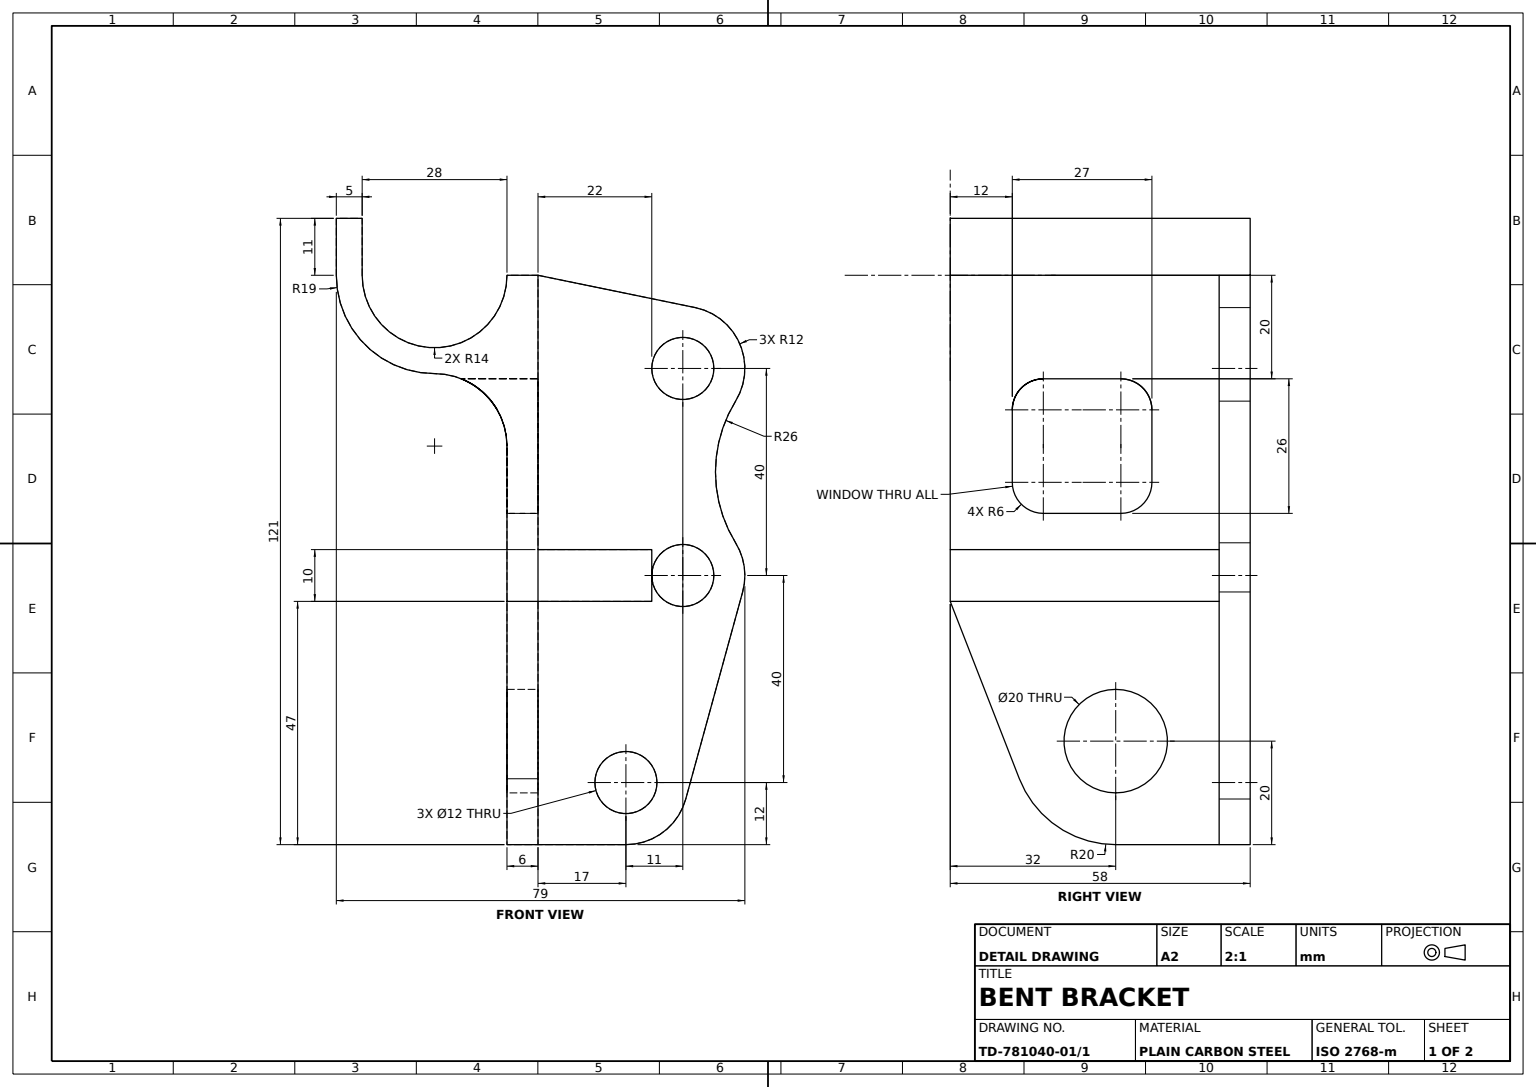
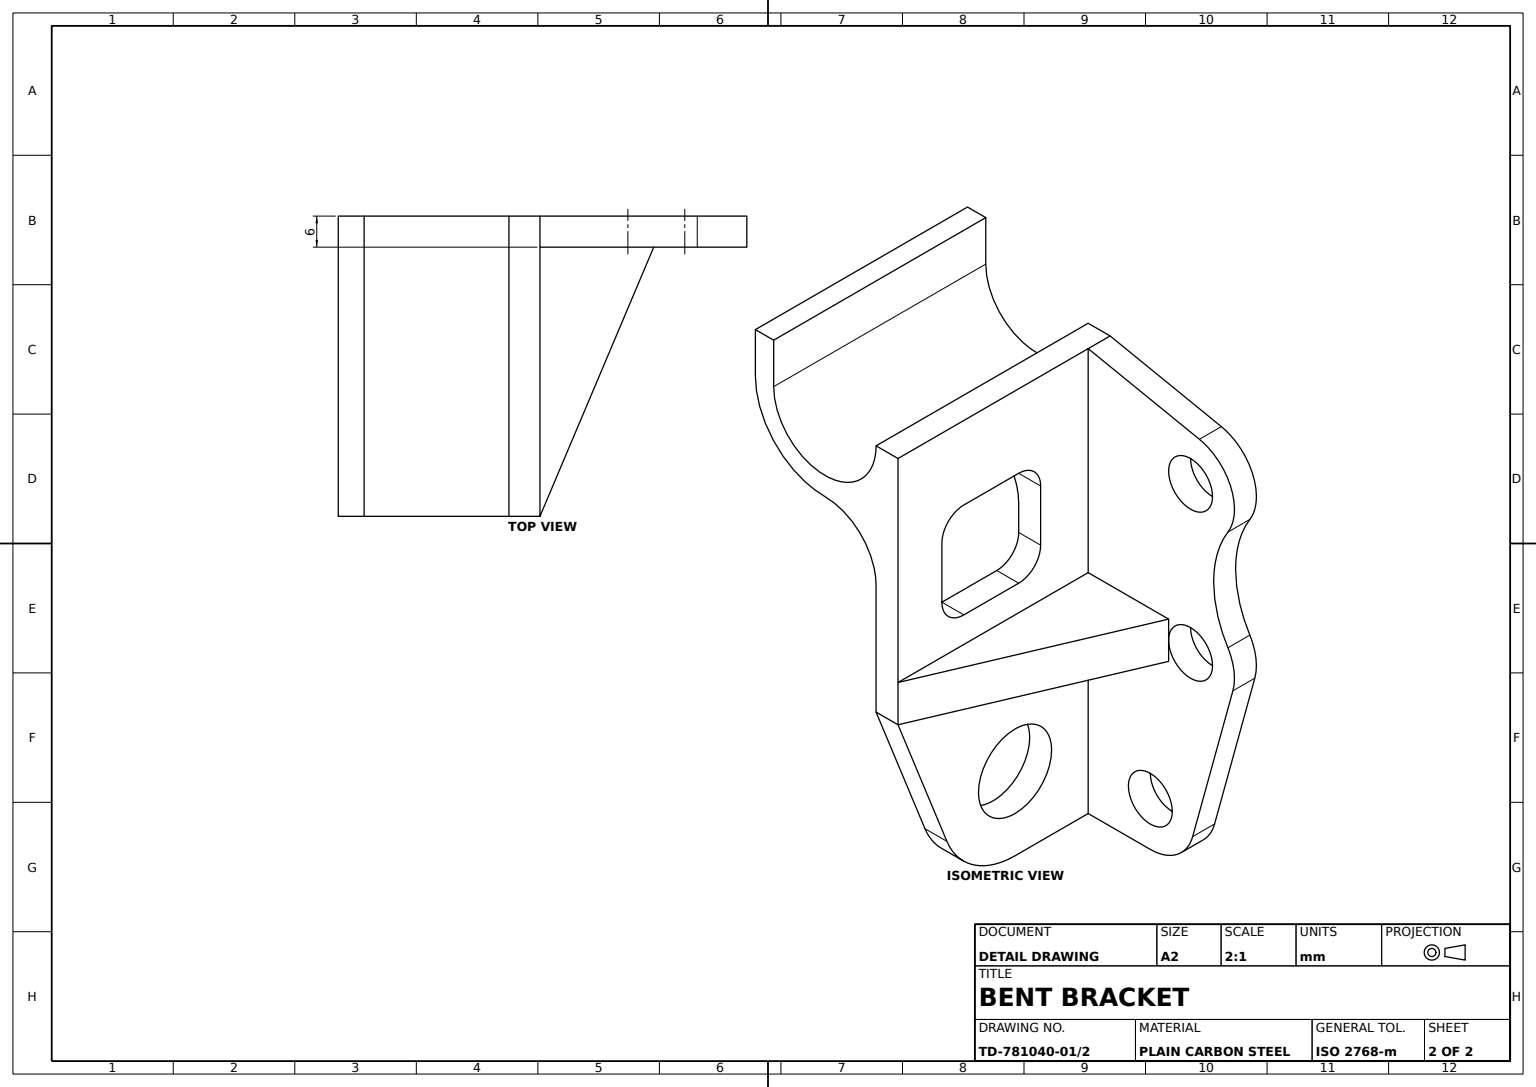
ISO-10303-21;
HEADER;
FILE_DESCRIPTION((''),'2;1');
FILE_NAME('','',(''),(''),'','','');
FILE_SCHEMA(('AUTOMOTIVE_DESIGN'));
ENDSEC;
DATA;
#1=APPLICATION_CONTEXT('');
#2=PRODUCT_CONTEXT('',#1,'mechanical');
#3=PRODUCT('','','',(#2));
#4=PRODUCT_DEFINITION_FORMATION('','',#3);
#5=PRODUCT_DEFINITION_CONTEXT('',#1,'design');
#6=PRODUCT_DEFINITION('','',#4,#5);
#7=PRODUCT_DEFINITION_SHAPE('','',#6);
#8=(LENGTH_UNIT()NAMED_UNIT(*)SI_UNIT(.MILLI.,.METRE.));
#9=(NAMED_UNIT(*)PLANE_ANGLE_UNIT()SI_UNIT($,.RADIAN.));
#10=(NAMED_UNIT(*)SI_UNIT($,.STERADIAN.)SOLID_ANGLE_UNIT());
#11=UNCERTAINTY_MEASURE_WITH_UNIT(LENGTH_MEASURE(1.E-05),#8,'distance_accuracy_value','');
#12=(GEOMETRIC_REPRESENTATION_CONTEXT(3)GLOBAL_UNCERTAINTY_ASSIGNED_CONTEXT((#11))GLOBAL_UNIT_ASSIGNED_CONTEXT((#8,#9,#10))REPRESENTATION_CONTEXT('',''));
#13=CARTESIAN_POINT('',(-39.,69.,-29.));
#14=VERTEX_POINT('',#13);
#15=CARTESIAN_POINT('',(-39.,58.,-29.));
#16=VERTEX_POINT('',#15);
#17=CARTESIAN_POINT('',(-39.,0.,-29.));
#18=DIRECTION('',(0.,-1.,0.));
#19=VECTOR('',#18,1000.);
#20=LINE('',#17,#19);
#21=EDGE_CURVE('',#14,#16,#20,.T.);
#22=ORIENTED_EDGE('',*,*,#21,.T.);
#23=CARTESIAN_POINT('',(-39.,58.,29.));
#24=VERTEX_POINT('',#23);
#25=DIRECTION('',(0.,0.,-1.));
#26=VECTOR('',#25,1000.);
#27=LINE('',#23,#26);
#28=EDGE_CURVE('',#24,#16,#27,.T.);
#29=ORIENTED_EDGE('',*,*,#28,.F.);
#30=CARTESIAN_POINT('',(-39.,69.,29.));
#31=VERTEX_POINT('',#30);
#32=CARTESIAN_POINT('',(-39.,0.,29.));
#33=LINE('',#32,#19);
#34=EDGE_CURVE('',#31,#24,#33,.T.);
#35=ORIENTED_EDGE('',*,*,#34,.F.);
#36=LINE('',#30,#26);
#37=EDGE_CURVE('',#31,#14,#36,.T.);
#38=ORIENTED_EDGE('',*,*,#37,.T.);
#39=EDGE_LOOP('',(#22,#29,#35,#38));
#40=FACE_OUTER_BOUND('',#39,.T.);
#41=DIRECTION('',(1.,0.,0.));
#42=DIRECTION('',(0.,1.,0.));
#43=AXIS2_PLACEMENT_3D('',#32,#41,#42);
#44=PLANE('',#43);
#45=ADVANCED_FACE('',(#40),#44,.F.);
#46=CARTESIAN_POINT('',(0.,-42.,-3.));
#47=VERTEX_POINT('',#46);
#48=CARTESIAN_POINT('',(0.,-22.,-3.));
#49=VERTEX_POINT('',#48);
#50=CARTESIAN_POINT('',(0.,-32.,-3.));
#51=AXIS2_PLACEMENT_3D('',#50,#41,#42);
#52=CIRCLE('',#51,10.);
#53=EDGE_CURVE('',#47,#49,#52,.T.);
#54=ORIENTED_EDGE('',*,*,#53,.F.);
#55=EDGE_CURVE('',#49,#47,#52,.T.);
#56=ORIENTED_EDGE('',*,*,#55,.F.);
#57=EDGE_LOOP('',(#54,#56));
#58=FACE_BOUND('',#57,.T.);
#59=CARTESIAN_POINT('',(0.,-39.268234,15.632573));
#60=VERTEX_POINT('',#59);
#61=CARTESIAN_POINT('',(0.,-52.,-3.));
#62=VERTEX_POINT('',#61);
#63=CIRCLE('',#51,20.);
#64=EDGE_CURVE('',#60,#62,#63,.T.);
#65=ORIENTED_EDGE('',*,*,#64,.T.);
#66=CARTESIAN_POINT('',(0.,-52.,-23.));
#67=VERTEX_POINT('',#66);
#68=CARTESIAN_POINT('',(0.,-52.,29.));
#69=LINE('',#68,#26);
#70=EDGE_CURVE('',#62,#67,#69,.T.);
#71=ORIENTED_EDGE('',*,*,#70,.T.);
#72=CARTESIAN_POINT('',(0.,-5.,-23.));
#73=VERTEX_POINT('',#72);
#74=CARTESIAN_POINT('',(0.,0.,-23.));
#75=LINE('',#74,#19);
#76=EDGE_CURVE('',#73,#67,#75,.T.);
#77=ORIENTED_EDGE('',*,*,#76,.F.);
#78=CARTESIAN_POINT('',(0.,-5.,29.));
#79=VERTEX_POINT('',#78);
#80=CARTESIAN_POINT('',(0.,-5.,0.));
#81=LINE('',#80,#26);
#82=EDGE_CURVE('',#79,#73,#81,.T.);
#83=ORIENTED_EDGE('',*,*,#82,.F.);
#84=CARTESIAN_POINT('',(0.,-10.478719,26.86285));
#85=DIRECTION('',(0.,0.931628639,0.363411721));
#86=VECTOR('',#85,1000.);
#87=LINE('',#84,#86);
#88=EDGE_CURVE('',#60,#79,#87,.T.);
#89=ORIENTED_EDGE('',*,*,#88,.F.);
#90=EDGE_LOOP('',(#65,#71,#77,#83,#89));
#91=FACE_OUTER_BOUND('',#90,.T.);
#92=CARTESIAN_POINT('',(0.,0.,29.));
#93=AXIS2_PLACEMENT_3D('',#92,#41,#42);
#94=PLANE('',#93);
#95=ADVANCED_FACE('',(#58,#91),#94,.T.);
#96=CARTESIAN_POINT('',(22.,0.,-23.));
#97=VERTEX_POINT('',#96);
#98=CARTESIAN_POINT('',(22.,-5.,-23.));
#99=VERTEX_POINT('',#98);
#100=CARTESIAN_POINT('',(22.,5.,-23.));
#101=LINE('',#100,#19);
#102=EDGE_CURVE('',#97,#99,#101,.T.);
#103=ORIENTED_EDGE('',*,*,#102,.F.);
#104=VERTEX_POINT('',#100);
#105=EDGE_CURVE('',#104,#97,#101,.T.);
#106=ORIENTED_EDGE('',*,*,#105,.F.);
#107=CARTESIAN_POINT('',(0.,5.,29.));
#108=VERTEX_POINT('',#107);
#109=CARTESIAN_POINT('',(10.406524,5.,4.40276));
#110=DIRECTION('',(0.389639991,0.,-0.920967251));
#111=VECTOR('',#110,1000.);
#112=LINE('',#109,#111);
#113=EDGE_CURVE('',#108,#104,#112,.T.);
#114=ORIENTED_EDGE('',*,*,#113,.F.);
#115=LINE('',#107,#19);
#116=EDGE_CURVE('',#108,#79,#115,.T.);
#117=ORIENTED_EDGE('',*,*,#116,.T.);
#118=CARTESIAN_POINT('',(10.406524,-5.,4.40276));
#119=LINE('',#118,#111);
#120=EDGE_CURVE('',#79,#99,#119,.T.);
#121=ORIENTED_EDGE('',*,*,#120,.T.);
#122=EDGE_LOOP('',(#103,#106,#114,#117,#121));
#123=FACE_OUTER_BOUND('',#122,.T.);
#124=DIRECTION('',(-0.920967251,0.,-0.389639991));
#125=DIRECTION('',(-0.389639991,0.,0.920967251));
#126=AXIS2_PLACEMENT_3D('',#109,#124,#125);
#127=PLANE('',#126);
#128=ADVANCED_FACE('',(#123),#127,.F.);
#129=ORIENTED_EDGE('',*,*,#64,.F.);
#130=CARTESIAN_POINT('',(-6.,-39.268234,15.632573));
#131=VERTEX_POINT('',#130);
#132=CARTESIAN_POINT('',(-39.001,-39.268234,15.632573));
#133=VECTOR('',#41,1000.);
#134=LINE('',#132,#133);
#135=EDGE_CURVE('',#131,#60,#134,.T.);
#136=ORIENTED_EDGE('',*,*,#135,.F.);
#137=CARTESIAN_POINT('',(-6.,-52.,-3.));
#138=VERTEX_POINT('',#137);
#139=CARTESIAN_POINT('',(-6.,-32.,-3.));
#140=DIRECTION('',(-1.,0.,0.));
#141=AXIS2_PLACEMENT_3D('',#139,#140,#42);
#142=CIRCLE('',#141,20.);
#143=EDGE_CURVE('',#138,#131,#142,.T.);
#144=ORIENTED_EDGE('',*,*,#143,.F.);
#145=CARTESIAN_POINT('',(-39.001,-52.,-3.));
#146=LINE('',#145,#133);
#147=EDGE_CURVE('',#138,#62,#146,.T.);
#148=ORIENTED_EDGE('',*,*,#147,.T.);
#149=EDGE_LOOP('',(#129,#136,#144,#148));
#150=FACE_OUTER_BOUND('',#149,.T.);
#151=CARTESIAN_POINT('',(-39.001,-32.,-3.));
#152=AXIS2_PLACEMENT_3D('',#151,#41,#42);
#153=CYLINDRICAL_SURFACE('',#152,20.);
#154=ADVANCED_FACE('',(#150),#153,.T.);
#155=CARTESIAN_POINT('',(30.413758,51.754734,-23.));
#156=VERTEX_POINT('',#155);
#157=CARTESIAN_POINT('',(30.413758,51.754734,-29.));
#158=VERTEX_POINT('',#157);
#159=LINE('',#155,#26);
#160=EDGE_CURVE('',#156,#158,#159,.T.);
#161=ORIENTED_EDGE('',*,*,#160,.F.);
#162=CARTESIAN_POINT('',(38.20347,33.684211,-23.));
#163=VERTEX_POINT('',#162);
#164=CARTESIAN_POINT('',(28.,40.,-23.));
#165=DIRECTION('',(0.,0.,1.));
#166=AXIS2_PLACEMENT_3D('',#164,#165,#41);
#167=CIRCLE('',#166,12.);
#168=EDGE_CURVE('',#163,#156,#167,.T.);
#169=ORIENTED_EDGE('',*,*,#168,.F.);
#170=CARTESIAN_POINT('',(38.20347,33.684211,-29.));
#171=VERTEX_POINT('',#170);
#172=LINE('',#162,#26);
#173=EDGE_CURVE('',#163,#171,#172,.T.);
#174=ORIENTED_EDGE('',*,*,#173,.T.);
#175=CARTESIAN_POINT('',(28.,40.,-29.));
#176=AXIS2_PLACEMENT_3D('',#175,#165,#41);
#177=CIRCLE('',#176,12.);
#178=EDGE_CURVE('',#171,#158,#177,.T.);
#179=ORIENTED_EDGE('',*,*,#178,.T.);
#180=EDGE_LOOP('',(#161,#169,#174,#179));
#181=FACE_OUTER_BOUND('',#180,.T.);
#182=AXIS2_PLACEMENT_3D('',#164,#25,#140);
#183=CYLINDRICAL_SURFACE('',#182,12.);
#184=ADVANCED_FACE('',(#181),#183,.T.);
#185=CARTESIAN_POINT('',(0.,58.,29.));
#186=VERTEX_POINT('',#185);
#187=CARTESIAN_POINT('',(-6.,58.,29.));
#188=VERTEX_POINT('',#187);
#189=VECTOR('',#140,1000.);
#190=LINE('',#185,#189);
#191=EDGE_CURVE('',#186,#188,#190,.T.);
#192=ORIENTED_EDGE('',*,*,#191,.F.);
#193=CARTESIAN_POINT('',(0.,58.,-23.));
#194=VERTEX_POINT('',#193);
#195=LINE('',#185,#26);
#196=EDGE_CURVE('',#186,#194,#195,.T.);
#197=ORIENTED_EDGE('',*,*,#196,.T.);
#198=CARTESIAN_POINT('',(0.,58.,-29.));
#199=VERTEX_POINT('',#198);
#200=LINE('',#193,#26);
#201=EDGE_CURVE('',#194,#199,#200,.T.);
#202=ORIENTED_EDGE('',*,*,#201,.T.);
#203=CARTESIAN_POINT('',(-6.,58.,-29.));
#204=VERTEX_POINT('',#203);
#205=LINE('',#198,#189);
#206=EDGE_CURVE('',#199,#204,#205,.T.);
#207=ORIENTED_EDGE('',*,*,#206,.T.);
#208=LINE('',#187,#26);
#209=EDGE_CURVE('',#188,#204,#208,.T.);
#210=ORIENTED_EDGE('',*,*,#209,.F.);
#211=EDGE_LOOP('',(#192,#197,#202,#207,#210));
#212=FACE_OUTER_BOUND('',#211,.T.);
#213=AXIS2_PLACEMENT_3D('',#185,#18,#41);
#214=PLANE('',#213);
#215=ADVANCED_FACE('',(#212),#214,.F.);
#216=CARTESIAN_POINT('',(-20.,39.,29.));
#217=VERTEX_POINT('',#216);
#218=CARTESIAN_POINT('',(-20.,58.,29.));
#219=AXIS2_PLACEMENT_3D('',#218,#165,#41);
#220=CIRCLE('',#219,19.);
#221=EDGE_CURVE('',#24,#217,#220,.T.);
#222=ORIENTED_EDGE('',*,*,#221,.F.);
#223=ORIENTED_EDGE('',*,*,#28,.T.);
#224=CARTESIAN_POINT('',(-20.,39.,-29.));
#225=VERTEX_POINT('',#224);
#226=CARTESIAN_POINT('',(-20.,58.,-29.));
#227=AXIS2_PLACEMENT_3D('',#226,#165,#41);
#228=CIRCLE('',#227,19.);
#229=EDGE_CURVE('',#16,#225,#228,.T.);
#230=ORIENTED_EDGE('',*,*,#229,.T.);
#231=VECTOR('',#165,1000.);
#232=LINE('',#216,#231);
#233=EDGE_CURVE('',#225,#217,#232,.T.);
#234=ORIENTED_EDGE('',*,*,#233,.T.);
#235=EDGE_LOOP('',(#222,#223,#230,#234));
#236=FACE_OUTER_BOUND('',#235,.T.);
#237=AXIS2_PLACEMENT_3D('',#218,#25,#140);
#238=CYLINDRICAL_SURFACE('',#237,19.);
#239=ADVANCED_FACE('',(#236),#238,.T.);
#240=ORIENTED_EDGE('',*,*,#173,.F.);
#241=CARTESIAN_POINT('',(34.310989,20.,-23.));
#242=VERTEX_POINT('',#241);
#243=CARTESIAN_POINT('',(60.310989,20.,-23.));
#244=AXIS2_PLACEMENT_3D('',#243,#165,#41);
#245=CIRCLE('',#244,26.);
#246=EDGE_CURVE('',#163,#242,#245,.T.);
#247=ORIENTED_EDGE('',*,*,#246,.T.);
#248=CARTESIAN_POINT('',(34.310989,20.,-29.));
#249=VERTEX_POINT('',#248);
#250=LINE('',#241,#26);
#251=EDGE_CURVE('',#242,#249,#250,.T.);
#252=ORIENTED_EDGE('',*,*,#251,.T.);
#253=CARTESIAN_POINT('',(60.310989,20.,-29.));
#254=AXIS2_PLACEMENT_3D('',#253,#165,#41);
#255=CIRCLE('',#254,26.);
#256=EDGE_CURVE('',#171,#249,#255,.T.);
#257=ORIENTED_EDGE('',*,*,#256,.F.);
#258=EDGE_LOOP('',(#240,#247,#252,#257));
#259=FACE_OUTER_BOUND('',#258,.T.);
#260=AXIS2_PLACEMENT_3D('',#243,#25,#140);
#261=CYLINDRICAL_SURFACE('',#260,26.);
#262=ADVANCED_FACE('',(#259),#261,.F.);
#263=ORIENTED_EDGE('',*,*,#120,.F.);
#264=ORIENTED_EDGE('',*,*,#82,.T.);
#265=LINE('',#72,#133);
#266=EDGE_CURVE('',#73,#99,#265,.T.);
#267=ORIENTED_EDGE('',*,*,#266,.T.);
#268=EDGE_LOOP('',(#263,#264,#267));
#269=FACE_OUTER_BOUND('',#268,.T.);
#270=AXIS2_PLACEMENT_3D('',#80,#42,#165);
#271=PLANE('',#270);
#272=ADVANCED_FACE('',(#269),#271,.F.);
#273=CARTESIAN_POINT('',(-6.,25.,-10.));
#274=VERTEX_POINT('',#273);
#275=CARTESIAN_POINT('',(-6.,25.,-29.));
#276=VERTEX_POINT('',#275);
#277=LINE('',#275,#26);
#278=EDGE_CURVE('',#274,#276,#277,.T.);
#279=ORIENTED_EDGE('',*,*,#278,.F.);
#280=CARTESIAN_POINT('',(-7.875644,32.,-10.));
#281=VERTEX_POINT('',#280);
#282=CARTESIAN_POINT('',(-20.,25.,-10.));
#283=AXIS2_PLACEMENT_3D('',#282,#25,#42);
#284=CIRCLE('',#283,14.);
#285=EDGE_CURVE('',#281,#274,#284,.T.);
#286=ORIENTED_EDGE('',*,*,#285,.F.);
#287=CARTESIAN_POINT('',(-14.803848,38.,-4.));
#288=VERTEX_POINT('',#287);
#289=CARTESIAN_POINT('',(-8.125276,32.432375,-10.));
#290=CARTESIAN_POINT('',(-8.392507,32.842114,-9.95397));
#291=CARTESIAN_POINT('',(-8.959761,33.622399,-9.790228));
#292=CARTESIAN_POINT('',(-9.259803,33.992885,-9.67229));
#293=CARTESIAN_POINT('',(-9.891376,34.697398,-9.373128));
#294=CARTESIAN_POINT('',(-10.216944,35.024563,-9.194584));
#295=CARTESIAN_POINT('',(-10.876753,35.628565,-8.792201));
#296=CARTESIAN_POINT('',(-11.212374,35.906825,-8.567711));
#297=CARTESIAN_POINT('',(-11.891238,36.420559,-8.072582));
#298=CARTESIAN_POINT('',(-12.236165,36.656785,-7.800557));
#299=CARTESIAN_POINT('',(-12.909548,37.078214,-7.215839));
#300=CARTESIAN_POINT('',(-13.240228,37.265008,-6.902669));
#301=CARTESIAN_POINT('',(-13.710866,37.509117,-6.384549));
#302=CARTESIAN_POINT('',(-13.864124,37.584761,-6.202612));
#303=CARTESIAN_POINT('',(-14.151016,37.720636,-5.820819));
#304=CARTESIAN_POINT('',(-14.284805,37.780965,-5.62123));
#305=CARTESIAN_POINT('',(-14.520473,37.883761,-5.195532));
#306=CARTESIAN_POINT('',(-14.621249,37.925746,-4.970388));
#307=CARTESIAN_POINT('',(-14.762952,37.983805,-4.50019));
#308=CARTESIAN_POINT('',(-14.803848,38.,-4.250793));
#309=B_SPLINE_CURVE_WITH_KNOTS('',3,(#280,#289,#290,#291,#292,#293,#294,#295,#296,#297,#298,#299,#300,#301,#302,#303,#304,#305,#306,#307,#308,#287),.UNSPECIFIED.,.F.,.F.,(4,2,2,2,2,2,2,2,2,2,4),(0.,0.001467721,0.002935441,0.004403162,0.005870883,0.007338603,0.008806324,0.009540185,0.010274045,0.011007905,0.011741766),.UNSPECIFIED.);
#310=EDGE_CURVE('',#281,#288,#309,.T.);
#311=ORIENTED_EDGE('',*,*,#310,.T.);
#312=CARTESIAN_POINT('',(-14.803848,38.,11.));
#313=VERTEX_POINT('',#312);
#314=CARTESIAN_POINT('',(-14.803848,38.,29.));
#315=LINE('',#314,#26);
#316=EDGE_CURVE('',#313,#288,#315,.T.);
#317=ORIENTED_EDGE('',*,*,#316,.F.);
#318=CARTESIAN_POINT('',(-7.875644,32.,17.));
#319=VERTEX_POINT('',#318);
#320=CARTESIAN_POINT('',(-14.803848,38.,11.251475));
#321=CARTESIAN_POINT('',(-14.764237,37.984323,11.494618));
#322=CARTESIAN_POINT('',(-14.657915,37.940773,11.849361));
#323=CARTESIAN_POINT('',(-14.614432,37.922788,11.966237));
#324=CARTESIAN_POINT('',(-14.516975,37.88174,12.190868));
#325=CARTESIAN_POINT('',(-14.462779,37.858587,12.299538));
#326=CARTESIAN_POINT('',(-14.287457,37.78214,12.616849));
#327=CARTESIAN_POINT('',(-14.153234,37.721658,12.817654));
#328=CARTESIAN_POINT('',(-13.865997,37.585677,13.200329));
#329=CARTESIAN_POINT('',(-13.714419,37.510893,13.380397));
#330=CARTESIAN_POINT('',(-13.245627,37.26794,13.897196));
#331=CARTESIAN_POINT('',(-12.91481,37.081351,14.211051));
#332=CARTESIAN_POINT('',(-12.238747,36.658555,14.798531));
#333=CARTESIAN_POINT('',(-11.896553,36.424247,15.06842));
#334=CARTESIAN_POINT('',(-11.220981,35.913665,15.561714));
#335=CARTESIAN_POINT('',(-10.886032,35.636525,15.786171));
#336=CARTESIAN_POINT('',(-10.390731,35.183907,16.088779));
#337=CARTESIAN_POINT('',(-10.226798,35.026854,16.183907));
#338=CARTESIAN_POINT('',(-9.901596,34.699253,16.361789));
#339=CARTESIAN_POINT('',(-9.74014,34.528414,16.444573));
#340=CARTESIAN_POINT('',(-9.26836,34.002974,16.668607));
#341=CARTESIAN_POINT('',(-8.967882,33.632936,16.787409));
#342=CARTESIAN_POINT('',(-8.396921,32.848806,16.95316));
#343=CARTESIAN_POINT('',(-8.124796,32.431543,17.));
#344=B_SPLINE_CURVE_WITH_KNOTS('',3,(#312,#320,#321,#322,#323,#324,#325,#326,#327,#328,#329,#330,#331,#332,#333,#334,#335,#336,#337,#338,#339,#340,#341,#342,#343,#318),.UNSPECIFIED.,.F.,.F.,(4,2,2,2,2,2,2,2,2,2,2,2,4),(0.,0.000740398,0.001110598,0.001480797,0.002221195,0.002961594,0.00444239,0.005923187,0.007403984,0.008144382,0.008884781,0.010365577,0.011846374),.UNSPECIFIED.);
#345=EDGE_CURVE('',#313,#319,#344,.T.);
#346=ORIENTED_EDGE('',*,*,#345,.T.);
#347=CARTESIAN_POINT('',(-6.,25.,17.));
#348=VERTEX_POINT('',#347);
#349=CARTESIAN_POINT('',(-20.,25.,17.));
#350=AXIS2_PLACEMENT_3D('',#349,#165,#18);
#351=CIRCLE('',#350,14.);
#352=EDGE_CURVE('',#348,#319,#351,.T.);
#353=ORIENTED_EDGE('',*,*,#352,.F.);
#354=CARTESIAN_POINT('',(-6.,25.,29.));
#355=VERTEX_POINT('',#354);
#356=EDGE_CURVE('',#355,#348,#277,.T.);
#357=ORIENTED_EDGE('',*,*,#356,.F.);
#358=CARTESIAN_POINT('',(-20.,25.,29.));
#359=AXIS2_PLACEMENT_3D('',#358,#25,#41);
#360=CIRCLE('',#359,14.);
#361=EDGE_CURVE('',#217,#355,#360,.T.);
#362=ORIENTED_EDGE('',*,*,#361,.F.);
#363=ORIENTED_EDGE('',*,*,#233,.F.);
#364=CARTESIAN_POINT('',(-20.,25.,-29.));
#365=AXIS2_PLACEMENT_3D('',#364,#165,#41);
#366=CIRCLE('',#365,14.);
#367=EDGE_CURVE('',#276,#225,#366,.T.);
#368=ORIENTED_EDGE('',*,*,#367,.F.);
#369=EDGE_LOOP('',(#279,#286,#311,#317,#346,#353,#357,#362,#363,#368));
#370=FACE_OUTER_BOUND('',#369,.T.);
#371=AXIS2_PLACEMENT_3D('',#358,#25,#140);
#372=CYLINDRICAL_SURFACE('',#371,14.);
#373=ADVANCED_FACE('',(#370),#372,.F.);
#374=ORIENTED_EDGE('',*,*,#356,.T.);
#375=CARTESIAN_POINT('',(-6.,18.,17.));
#376=VERTEX_POINT('',#375);
#377=CARTESIAN_POINT('',(-6.,38.,17.));
#378=VECTOR('',#42,1000.);
#379=LINE('',#377,#378);
#380=EDGE_CURVE('',#376,#348,#379,.T.);
#381=ORIENTED_EDGE('',*,*,#380,.F.);
#382=CARTESIAN_POINT('',(-6.,12.,11.));
#383=VERTEX_POINT('',#382);
#384=CARTESIAN_POINT('',(-6.,18.,11.));
#385=AXIS2_PLACEMENT_3D('',#384,#41,#42);
#386=CIRCLE('',#385,6.);
#387=EDGE_CURVE('',#376,#383,#386,.T.);
#388=ORIENTED_EDGE('',*,*,#387,.T.);
#389=CARTESIAN_POINT('',(-6.,12.,-4.));
#390=VERTEX_POINT('',#389);
#391=CARTESIAN_POINT('',(-6.,12.,17.));
#392=LINE('',#391,#231);
#393=EDGE_CURVE('',#390,#383,#392,.T.);
#394=ORIENTED_EDGE('',*,*,#393,.F.);
#395=CARTESIAN_POINT('',(-6.,18.,-10.));
#396=VERTEX_POINT('',#395);
#397=CARTESIAN_POINT('',(-6.,18.,-4.));
#398=AXIS2_PLACEMENT_3D('',#397,#41,#42);
#399=CIRCLE('',#398,6.);
#400=EDGE_CURVE('',#390,#396,#399,.T.);
#401=ORIENTED_EDGE('',*,*,#400,.T.);
#402=CARTESIAN_POINT('',(-6.,38.,-10.));
#403=LINE('',#402,#19);
#404=EDGE_CURVE('',#274,#396,#403,.T.);
#405=ORIENTED_EDGE('',*,*,#404,.F.);
#406=ORIENTED_EDGE('',*,*,#278,.T.);
#407=CARTESIAN_POINT('',(-6.,-52.,-29.));
#408=VERTEX_POINT('',#407);
#409=CARTESIAN_POINT('',(-6.,0.,-29.));
#410=LINE('',#409,#19);
#411=EDGE_CURVE('',#276,#408,#410,.T.);
#412=ORIENTED_EDGE('',*,*,#411,.T.);
#413=CARTESIAN_POINT('',(-6.,-52.,29.));
#414=LINE('',#413,#26);
#415=EDGE_CURVE('',#138,#408,#414,.T.);
#416=ORIENTED_EDGE('',*,*,#415,.F.);
#417=ORIENTED_EDGE('',*,*,#143,.T.);
#418=CARTESIAN_POINT('',(-6.,-5.,29.));
#419=VERTEX_POINT('',#418);
#420=CARTESIAN_POINT('',(-6.,-10.478719,26.86285));
#421=DIRECTION('',(0.,-0.931628639,-0.363411721));
#422=VECTOR('',#421,1000.);
#423=LINE('',#420,#422);
#424=EDGE_CURVE('',#419,#131,#423,.T.);
#425=ORIENTED_EDGE('',*,*,#424,.F.);
#426=CARTESIAN_POINT('',(-6.,0.,29.));
#427=LINE('',#426,#19);
#428=EDGE_CURVE('',#355,#419,#427,.T.);
#429=ORIENTED_EDGE('',*,*,#428,.F.);
#430=EDGE_LOOP('',(#374,#381,#388,#394,#401,#405,#406,#412,#416,#417,#425,#429));
#431=FACE_OUTER_BOUND('',#430,.T.);
#432=CARTESIAN_POINT('',(-6.,-22.,-3.));
#433=VERTEX_POINT('',#432);
#434=CARTESIAN_POINT('',(-6.,-42.,-3.));
#435=VERTEX_POINT('',#434);
#436=CIRCLE('',#141,10.);
#437=EDGE_CURVE('',#433,#435,#436,.T.);
#438=ORIENTED_EDGE('',*,*,#437,.F.);
#439=EDGE_CURVE('',#435,#433,#436,.T.);
#440=ORIENTED_EDGE('',*,*,#439,.F.);
#441=EDGE_LOOP('',(#438,#440));
#442=FACE_BOUND('',#441,.T.);
#443=AXIS2_PLACEMENT_3D('',#426,#41,#42);
#444=PLANE('',#443);
#445=ADVANCED_FACE('',(#431,#442),#444,.F.);
#446=CARTESIAN_POINT('',(39.570465,-3.181878,-23.));
#447=VERTEX_POINT('',#446);
#448=CARTESIAN_POINT('',(39.570465,-3.181878,-29.));
#449=VERTEX_POINT('',#448);
#450=LINE('',#446,#26);
#451=EDGE_CURVE('',#447,#449,#450,.T.);
#452=ORIENTED_EDGE('',*,*,#451,.F.);
#453=CARTESIAN_POINT('',(28.570465,-43.181878,-23.));
#454=VERTEX_POINT('',#453);
#455=CARTESIAN_POINT('',(37.601842,-10.340507,-23.));
#456=DIRECTION('',(0.265156483,0.964205393,0.));
#457=VECTOR('',#456,1000.);
#458=LINE('',#455,#457);
#459=EDGE_CURVE('',#454,#447,#458,.T.);
#460=ORIENTED_EDGE('',*,*,#459,.F.);
#461=CARTESIAN_POINT('',(28.570465,-43.181878,-29.));
#462=VERTEX_POINT('',#461);
#463=LINE('',#453,#26);
#464=EDGE_CURVE('',#454,#462,#463,.T.);
#465=ORIENTED_EDGE('',*,*,#464,.T.);
#466=CARTESIAN_POINT('',(37.601842,-10.340507,-29.));
#467=LINE('',#466,#457);
#468=EDGE_CURVE('',#462,#449,#467,.T.);
#469=ORIENTED_EDGE('',*,*,#468,.T.);
#470=EDGE_LOOP('',(#452,#460,#465,#469));
#471=FACE_OUTER_BOUND('',#470,.T.);
#472=DIRECTION('',(-0.964205393,0.265156483,0.));
#473=DIRECTION('',(-0.265156483,-0.964205393,0.));
#474=AXIS2_PLACEMENT_3D('',#455,#472,#473);
#475=PLANE('',#474);
#476=ADVANCED_FACE('',(#471),#475,.F.);
#477=CARTESIAN_POINT('',(0.,5.,-23.));
#478=VERTEX_POINT('',#477);
#479=CARTESIAN_POINT('',(0.,5.,0.));
#480=LINE('',#479,#26);
#481=EDGE_CURVE('',#108,#478,#480,.T.);
#482=ORIENTED_EDGE('',*,*,#481,.F.);
#483=ORIENTED_EDGE('',*,*,#113,.T.);
#484=LINE('',#477,#133);
#485=EDGE_CURVE('',#478,#104,#484,.T.);
#486=ORIENTED_EDGE('',*,*,#485,.F.);
#487=EDGE_LOOP('',(#482,#483,#486));
#488=FACE_OUTER_BOUND('',#487,.T.);
#489=AXIS2_PLACEMENT_3D('',#479,#42,#165);
#490=PLANE('',#489);
#491=ADVANCED_FACE('',(#488),#490,.T.);
#492=CARTESIAN_POINT('',(11.,-40.,-23.));
#493=VERTEX_POINT('',#492);
#494=CARTESIAN_POINT('',(23.,-40.,-23.));
#495=VERTEX_POINT('',#494);
#496=CARTESIAN_POINT('',(17.,-40.,-23.));
#497=AXIS2_PLACEMENT_3D('',#496,#165,#41);
#498=CIRCLE('',#497,6.);
#499=EDGE_CURVE('',#493,#495,#498,.T.);
#500=ORIENTED_EDGE('',*,*,#499,.T.);
#501=CARTESIAN_POINT('',(23.,-40.,-29.));
#502=VERTEX_POINT('',#501);
#503=LINE('',#494,#26);
#504=EDGE_CURVE('',#495,#502,#503,.T.);
#505=ORIENTED_EDGE('',*,*,#504,.T.);
#506=CARTESIAN_POINT('',(11.,-40.,-29.));
#507=VERTEX_POINT('',#506);
#508=CARTESIAN_POINT('',(17.,-40.,-29.));
#509=AXIS2_PLACEMENT_3D('',#508,#165,#41);
#510=CIRCLE('',#509,6.);
#511=EDGE_CURVE('',#507,#502,#510,.T.);
#512=ORIENTED_EDGE('',*,*,#511,.F.);
#513=LINE('',#492,#26);
#514=EDGE_CURVE('',#493,#507,#513,.T.);
#515=ORIENTED_EDGE('',*,*,#514,.F.);
#516=EDGE_LOOP('',(#500,#505,#512,#515));
#517=FACE_OUTER_BOUND('',#516,.T.);
#518=AXIS2_PLACEMENT_3D('',#496,#25,#140);
#519=CYLINDRICAL_SURFACE('',#518,6.);
#520=ADVANCED_FACE('',(#517),#519,.F.);
#521=CARTESIAN_POINT('',(-34.,58.,29.));
#522=VERTEX_POINT('',#521);
#523=CARTESIAN_POINT('',(-34.,69.,29.));
#524=VERTEX_POINT('',#523);
#525=CARTESIAN_POINT('',(-34.,0.,29.));
#526=LINE('',#525,#378);
#527=EDGE_CURVE('',#522,#524,#526,.T.);
#528=ORIENTED_EDGE('',*,*,#527,.F.);
#529=CARTESIAN_POINT('',(-34.,58.,-29.));
#530=VERTEX_POINT('',#529);
#531=LINE('',#521,#26);
#532=EDGE_CURVE('',#522,#530,#531,.T.);
#533=ORIENTED_EDGE('',*,*,#532,.T.);
#534=CARTESIAN_POINT('',(-34.,69.,-29.));
#535=VERTEX_POINT('',#534);
#536=CARTESIAN_POINT('',(-34.,0.,-29.));
#537=LINE('',#536,#378);
#538=EDGE_CURVE('',#530,#535,#537,.T.);
#539=ORIENTED_EDGE('',*,*,#538,.T.);
#540=LINE('',#523,#26);
#541=EDGE_CURVE('',#524,#535,#540,.T.);
#542=ORIENTED_EDGE('',*,*,#541,.F.);
#543=EDGE_LOOP('',(#528,#533,#539,#542));
#544=FACE_OUTER_BOUND('',#543,.T.);
#545=AXIS2_PLACEMENT_3D('',#525,#140,#165);
#546=PLANE('',#545);
#547=ADVANCED_FACE('',(#544),#546,.F.);
#548=CARTESIAN_POINT('',(0.,38.,-4.));
#549=VERTEX_POINT('',#548);
#550=CARTESIAN_POINT('',(0.,38.,11.));
#551=VERTEX_POINT('',#550);
#552=CARTESIAN_POINT('',(0.,38.,17.));
#553=LINE('',#552,#231);
#554=EDGE_CURVE('',#549,#551,#553,.T.);
#555=ORIENTED_EDGE('',*,*,#554,.T.);
#556=LINE('',#312,#189);
#557=EDGE_CURVE('',#551,#313,#556,.T.);
#558=ORIENTED_EDGE('',*,*,#557,.T.);
#559=ORIENTED_EDGE('',*,*,#316,.T.);
#560=LINE('',#548,#133);
#561=EDGE_CURVE('',#288,#549,#560,.T.);
#562=ORIENTED_EDGE('',*,*,#561,.T.);
#563=EDGE_LOOP('',(#555,#558,#559,#562));
#564=FACE_OUTER_BOUND('',#563,.T.);
#565=CARTESIAN_POINT('',(-39.001,38.,17.));
#566=AXIS2_PLACEMENT_3D('',#565,#42,#140);
#567=PLANE('',#566);
#568=ADVANCED_FACE('',(#564),#567,.F.);
#569=CARTESIAN_POINT('',(38.20347,6.315789,-23.));
#570=VERTEX_POINT('',#569);
#571=CARTESIAN_POINT('',(28.,0.,-23.));
#572=AXIS2_PLACEMENT_3D('',#571,#165,#41);
#573=CIRCLE('',#572,12.);
#574=EDGE_CURVE('',#447,#570,#573,.T.);
#575=ORIENTED_EDGE('',*,*,#574,.F.);
#576=ORIENTED_EDGE('',*,*,#451,.T.);
#577=CARTESIAN_POINT('',(38.20347,6.315789,-29.));
#578=VERTEX_POINT('',#577);
#579=CARTESIAN_POINT('',(28.,0.,-29.));
#580=AXIS2_PLACEMENT_3D('',#579,#165,#41);
#581=CIRCLE('',#580,12.);
#582=EDGE_CURVE('',#449,#578,#581,.T.);
#583=ORIENTED_EDGE('',*,*,#582,.T.);
#584=LINE('',#569,#26);
#585=EDGE_CURVE('',#570,#578,#584,.T.);
#586=ORIENTED_EDGE('',*,*,#585,.F.);
#587=EDGE_LOOP('',(#575,#576,#583,#586));
#588=FACE_OUTER_BOUND('',#587,.T.);
#589=AXIS2_PLACEMENT_3D('',#571,#25,#140);
#590=CYLINDRICAL_SURFACE('',#589,12.);
#591=ADVANCED_FACE('',(#588),#590,.T.);
#592=ORIENTED_EDGE('',*,*,#459,.T.);
#593=ORIENTED_EDGE('',*,*,#574,.T.);
#594=EDGE_CURVE('',#242,#570,#245,.T.);
#595=ORIENTED_EDGE('',*,*,#594,.F.);
#596=ORIENTED_EDGE('',*,*,#246,.F.);
#597=ORIENTED_EDGE('',*,*,#168,.T.);
#598=CARTESIAN_POINT('',(11.428046,55.653326,-23.));
#599=DIRECTION('',(-0.979561176,0.20114647,0.));
#600=VECTOR('',#599,1000.);
#601=LINE('',#598,#600);
#602=EDGE_CURVE('',#156,#194,#601,.T.);
#603=ORIENTED_EDGE('',*,*,#602,.T.);
#604=EDGE_CURVE('',#194,#478,#75,.T.);
#605=ORIENTED_EDGE('',*,*,#604,.T.);
#606=ORIENTED_EDGE('',*,*,#485,.T.);
#607=ORIENTED_EDGE('',*,*,#105,.T.);
#608=CARTESIAN_POINT('',(34.,0.,-23.));
#609=VERTEX_POINT('',#608);
#610=CIRCLE('',#572,6.);
#611=EDGE_CURVE('',#609,#97,#610,.T.);
#612=ORIENTED_EDGE('',*,*,#611,.F.);
#613=EDGE_CURVE('',#97,#609,#610,.T.);
#614=ORIENTED_EDGE('',*,*,#613,.F.);
#615=ORIENTED_EDGE('',*,*,#102,.T.);
#616=ORIENTED_EDGE('',*,*,#266,.F.);
#617=ORIENTED_EDGE('',*,*,#76,.T.);
#618=CARTESIAN_POINT('',(17.,-52.,-23.));
#619=VERTEX_POINT('',#618);
#620=LINE('',#66,#133);
#621=EDGE_CURVE('',#67,#619,#620,.T.);
#622=ORIENTED_EDGE('',*,*,#621,.T.);
#623=CIRCLE('',#497,12.);
#624=EDGE_CURVE('',#619,#454,#623,.T.);
#625=ORIENTED_EDGE('',*,*,#624,.T.);
#626=EDGE_LOOP('',(#592,#593,#595,#596,#597,#603,#605,#606,#607,#612,#614,#615,#616,#617,#622,#625));
#627=FACE_OUTER_BOUND('',#626,.T.);
#628=CARTESIAN_POINT('',(34.,40.,-23.));
#629=VERTEX_POINT('',#628);
#630=CARTESIAN_POINT('',(22.,40.,-23.));
#631=VERTEX_POINT('',#630);
#632=CIRCLE('',#166,6.);
#633=EDGE_CURVE('',#629,#631,#632,.T.);
#634=ORIENTED_EDGE('',*,*,#633,.F.);
#635=EDGE_CURVE('',#631,#629,#632,.T.);
#636=ORIENTED_EDGE('',*,*,#635,.F.);
#637=EDGE_LOOP('',(#634,#636));
#638=FACE_BOUND('',#637,.T.);
#639=EDGE_CURVE('',#495,#493,#498,.T.);
#640=ORIENTED_EDGE('',*,*,#639,.F.);
#641=ORIENTED_EDGE('',*,*,#499,.F.);
#642=EDGE_LOOP('',(#640,#641));
#643=FACE_BOUND('',#642,.T.);
#644=PLANE('',#244);
#645=ADVANCED_FACE('',(#627,#638,#643),#644,.T.);
#646=CARTESIAN_POINT('',(0.,12.,11.));
#647=VERTEX_POINT('',#646);
#648=LINE('',#646,#133);
#649=EDGE_CURVE('',#383,#647,#648,.T.);
#650=ORIENTED_EDGE('',*,*,#649,.F.);
#651=ORIENTED_EDGE('',*,*,#387,.F.);
#652=CARTESIAN_POINT('',(0.,18.,17.));
#653=VERTEX_POINT('',#652);
#654=LINE('',#375,#189);
#655=EDGE_CURVE('',#653,#376,#654,.T.);
#656=ORIENTED_EDGE('',*,*,#655,.F.);
#657=CARTESIAN_POINT('',(0.,18.,11.));
#658=AXIS2_PLACEMENT_3D('',#657,#140,#42);
#659=CIRCLE('',#658,6.);
#660=EDGE_CURVE('',#647,#653,#659,.T.);
#661=ORIENTED_EDGE('',*,*,#660,.F.);
#662=EDGE_LOOP('',(#650,#651,#656,#661));
#663=FACE_OUTER_BOUND('',#662,.T.);
#664=CARTESIAN_POINT('',(-39.001,18.,11.));
#665=AXIS2_PLACEMENT_3D('',#664,#140,#18);
#666=CYLINDRICAL_SURFACE('',#665,6.);
#667=ADVANCED_FACE('',(#663),#666,.F.);
#668=ORIENTED_EDGE('',*,*,#639,.T.);
#669=ORIENTED_EDGE('',*,*,#514,.T.);
#670=EDGE_CURVE('',#502,#507,#510,.T.);
#671=ORIENTED_EDGE('',*,*,#670,.F.);
#672=ORIENTED_EDGE('',*,*,#504,.F.);
#673=EDGE_LOOP('',(#668,#669,#671,#672));
#674=FACE_OUTER_BOUND('',#673,.T.);
#675=ADVANCED_FACE('',(#674),#519,.F.);
#676=ORIENTED_EDGE('',*,*,#585,.T.);
#677=EDGE_CURVE('',#249,#578,#255,.T.);
#678=ORIENTED_EDGE('',*,*,#677,.F.);
#679=ORIENTED_EDGE('',*,*,#251,.F.);
#680=ORIENTED_EDGE('',*,*,#594,.T.);
#681=EDGE_LOOP('',(#676,#678,#679,#680));
#682=FACE_OUTER_BOUND('',#681,.T.);
#683=ADVANCED_FACE('',(#682),#261,.F.);
#684=ORIENTED_EDGE('',*,*,#209,.T.);
#685=CIRCLE('',#227,14.);
#686=EDGE_CURVE('',#530,#204,#685,.T.);
#687=ORIENTED_EDGE('',*,*,#686,.F.);
#688=ORIENTED_EDGE('',*,*,#532,.F.);
#689=CIRCLE('',#219,14.);
#690=EDGE_CURVE('',#522,#188,#689,.T.);
#691=ORIENTED_EDGE('',*,*,#690,.T.);
#692=EDGE_LOOP('',(#684,#687,#688,#691));
#693=FACE_OUTER_BOUND('',#692,.T.);
#694=CYLINDRICAL_SURFACE('',#237,14.);
#695=ADVANCED_FACE('',(#693),#694,.F.);
#696=ORIENTED_EDGE('',*,*,#135,.T.);
#697=ORIENTED_EDGE('',*,*,#88,.T.);
#698=CARTESIAN_POINT('',(-39.001,-5.,29.));
#699=LINE('',#698,#133);
#700=EDGE_CURVE('',#419,#79,#699,.T.);
#701=ORIENTED_EDGE('',*,*,#700,.F.);
#702=ORIENTED_EDGE('',*,*,#424,.T.);
#703=EDGE_LOOP('',(#696,#697,#701,#702));
#704=FACE_OUTER_BOUND('',#703,.T.);
#705=CARTESIAN_POINT('',(-39.001,-10.478719,26.86285));
#706=DIRECTION('',(0.,0.363411721,-0.931628639));
#707=AXIS2_PLACEMENT_3D('',#705,#706,#85);
#708=PLANE('',#707);
#709=ADVANCED_FACE('',(#704),#708,.F.);
#710=ORIENTED_EDGE('',*,*,#147,.F.);
#711=ORIENTED_EDGE('',*,*,#415,.T.);
#712=CARTESIAN_POINT('',(17.,-52.,-29.));
#713=VERTEX_POINT('',#712);
#714=CARTESIAN_POINT('',(0.,-52.,-29.));
#715=LINE('',#714,#133);
#716=EDGE_CURVE('',#408,#713,#715,.T.);
#717=ORIENTED_EDGE('',*,*,#716,.T.);
#718=LINE('',#618,#26);
#719=EDGE_CURVE('',#619,#713,#718,.T.);
#720=ORIENTED_EDGE('',*,*,#719,.F.);
#721=ORIENTED_EDGE('',*,*,#621,.F.);
#722=ORIENTED_EDGE('',*,*,#70,.F.);
#723=EDGE_LOOP('',(#710,#711,#717,#720,#721,#722));
#724=FACE_OUTER_BOUND('',#723,.T.);
#725=AXIS2_PLACEMENT_3D('',#68,#42,#165);
#726=PLANE('',#725);
#727=ADVANCED_FACE('',(#724),#726,.F.);
#728=ORIENTED_EDGE('',*,*,#719,.T.);
#729=CIRCLE('',#509,12.);
#730=EDGE_CURVE('',#713,#462,#729,.T.);
#731=ORIENTED_EDGE('',*,*,#730,.T.);
#732=ORIENTED_EDGE('',*,*,#464,.F.);
#733=ORIENTED_EDGE('',*,*,#624,.F.);
#734=EDGE_LOOP('',(#728,#731,#732,#733));
#735=FACE_OUTER_BOUND('',#734,.T.);
#736=CYLINDRICAL_SURFACE('',#518,12.);
#737=ADVANCED_FACE('',(#735),#736,.T.);
#738=CARTESIAN_POINT('',(22.,40.,-29.));
#739=VERTEX_POINT('',#738);
#740=LINE('',#630,#26);
#741=EDGE_CURVE('',#631,#739,#740,.T.);
#742=ORIENTED_EDGE('',*,*,#741,.T.);
#743=CARTESIAN_POINT('',(34.,40.,-29.));
#744=VERTEX_POINT('',#743);
#745=CIRCLE('',#176,6.);
#746=EDGE_CURVE('',#744,#739,#745,.T.);
#747=ORIENTED_EDGE('',*,*,#746,.F.);
#748=LINE('',#628,#26);
#749=EDGE_CURVE('',#629,#744,#748,.T.);
#750=ORIENTED_EDGE('',*,*,#749,.F.);
#751=ORIENTED_EDGE('',*,*,#633,.T.);
#752=EDGE_LOOP('',(#742,#747,#750,#751));
#753=FACE_OUTER_BOUND('',#752,.T.);
#754=CYLINDRICAL_SURFACE('',#182,6.);
#755=ADVANCED_FACE('',(#753),#754,.F.);
#756=CARTESIAN_POINT('',(0.,18.,-10.));
#757=VERTEX_POINT('',#756);
#758=LINE('',#756,#133);
#759=EDGE_CURVE('',#396,#757,#758,.T.);
#760=ORIENTED_EDGE('',*,*,#759,.T.);
#761=CARTESIAN_POINT('',(0.,32.,-10.));
#762=VERTEX_POINT('',#761);
#763=CARTESIAN_POINT('',(0.,38.,-10.));
#764=LINE('',#763,#378);
#765=EDGE_CURVE('',#757,#762,#764,.T.);
#766=ORIENTED_EDGE('',*,*,#765,.T.);
#767=CARTESIAN_POINT('',(-14.803848,32.,-10.));
#768=LINE('',#767,#189);
#769=EDGE_CURVE('',#762,#281,#768,.T.);
#770=ORIENTED_EDGE('',*,*,#769,.T.);
#771=ORIENTED_EDGE('',*,*,#285,.T.);
#772=ORIENTED_EDGE('',*,*,#404,.T.);
#773=EDGE_LOOP('',(#760,#766,#770,#771,#772));
#774=FACE_OUTER_BOUND('',#773,.T.);
#775=CARTESIAN_POINT('',(-39.001,38.,-10.));
#776=AXIS2_PLACEMENT_3D('',#775,#25,#42);
#777=PLANE('',#776);
#778=ADVANCED_FACE('',(#774),#777,.F.);
#779=ORIENTED_EDGE('',*,*,#613,.T.);
#780=CARTESIAN_POINT('',(34.,0.,-29.));
#781=VERTEX_POINT('',#780);
#782=LINE('',#608,#26);
#783=EDGE_CURVE('',#609,#781,#782,.T.);
#784=ORIENTED_EDGE('',*,*,#783,.T.);
#785=CARTESIAN_POINT('',(22.,0.,-29.));
#786=VERTEX_POINT('',#785);
#787=CIRCLE('',#580,6.);
#788=EDGE_CURVE('',#786,#781,#787,.T.);
#789=ORIENTED_EDGE('',*,*,#788,.F.);
#790=LINE('',#96,#26);
#791=EDGE_CURVE('',#97,#786,#790,.T.);
#792=ORIENTED_EDGE('',*,*,#791,.F.);
#793=EDGE_LOOP('',(#779,#784,#789,#792));
#794=FACE_OUTER_BOUND('',#793,.T.);
#795=CYLINDRICAL_SURFACE('',#589,6.);
#796=ADVANCED_FACE('',(#794),#795,.F.);
#797=ORIENTED_EDGE('',*,*,#201,.F.);
#798=ORIENTED_EDGE('',*,*,#602,.F.);
#799=ORIENTED_EDGE('',*,*,#160,.T.);
#800=CARTESIAN_POINT('',(11.428046,55.653326,-29.));
#801=LINE('',#800,#600);
#802=EDGE_CURVE('',#158,#199,#801,.T.);
#803=ORIENTED_EDGE('',*,*,#802,.T.);
#804=EDGE_LOOP('',(#797,#798,#799,#803));
#805=FACE_OUTER_BOUND('',#804,.T.);
#806=DIRECTION('',(-0.20114647,-0.979561176,0.));
#807=DIRECTION('',(0.979561176,-0.20114647,0.));
#808=AXIS2_PLACEMENT_3D('',#598,#806,#807);
#809=PLANE('',#808);
#810=ADVANCED_FACE('',(#805),#809,.F.);
#811=ORIENTED_EDGE('',*,*,#649,.T.);
#812=CARTESIAN_POINT('',(0.,12.,-4.));
#813=VERTEX_POINT('',#812);
#814=CARTESIAN_POINT('',(0.,12.,17.));
#815=LINE('',#814,#26);
#816=EDGE_CURVE('',#647,#813,#815,.T.);
#817=ORIENTED_EDGE('',*,*,#816,.T.);
#818=LINE('',#389,#189);
#819=EDGE_CURVE('',#813,#390,#818,.T.);
#820=ORIENTED_EDGE('',*,*,#819,.T.);
#821=ORIENTED_EDGE('',*,*,#393,.T.);
#822=EDGE_LOOP('',(#811,#817,#820,#821));
#823=FACE_OUTER_BOUND('',#822,.T.);
#824=CARTESIAN_POINT('',(-39.001,12.,17.));
#825=AXIS2_PLACEMENT_3D('',#824,#18,#41);
#826=PLANE('',#825);
#827=ADVANCED_FACE('',(#823),#826,.F.);
#828=ORIENTED_EDGE('',*,*,#635,.T.);
#829=ORIENTED_EDGE('',*,*,#749,.T.);
#830=EDGE_CURVE('',#739,#744,#745,.T.);
#831=ORIENTED_EDGE('',*,*,#830,.F.);
#832=ORIENTED_EDGE('',*,*,#741,.F.);
#833=EDGE_LOOP('',(#828,#829,#831,#832));
#834=FACE_OUTER_BOUND('',#833,.T.);
#835=ADVANCED_FACE('',(#834),#754,.F.);
#836=ORIENTED_EDGE('',*,*,#310,.F.);
#837=ORIENTED_EDGE('',*,*,#769,.F.);
#838=CARTESIAN_POINT('',(0.,32.,-4.));
#839=AXIS2_PLACEMENT_3D('',#838,#140,#42);
#840=CIRCLE('',#839,6.);
#841=EDGE_CURVE('',#549,#762,#840,.T.);
#842=ORIENTED_EDGE('',*,*,#841,.F.);
#843=ORIENTED_EDGE('',*,*,#561,.F.);
#844=EDGE_LOOP('',(#836,#837,#842,#843));
#845=FACE_OUTER_BOUND('',#844,.T.);
#846=CARTESIAN_POINT('',(-39.001,32.,-4.));
#847=AXIS2_PLACEMENT_3D('',#846,#140,#18);
#848=CYLINDRICAL_SURFACE('',#847,6.);
#849=ADVANCED_FACE('',(#845),#848,.F.);
#850=CARTESIAN_POINT('',(0.,69.,-29.));
#851=LINE('',#850,#189);
#852=EDGE_CURVE('',#535,#14,#851,.T.);
#853=ORIENTED_EDGE('',*,*,#852,.T.);
#854=ORIENTED_EDGE('',*,*,#37,.F.);
#855=CARTESIAN_POINT('',(0.,69.,29.));
#856=LINE('',#855,#189);
#857=EDGE_CURVE('',#524,#31,#856,.T.);
#858=ORIENTED_EDGE('',*,*,#857,.F.);
#859=ORIENTED_EDGE('',*,*,#541,.T.);
#860=EDGE_LOOP('',(#853,#854,#858,#859));
#861=FACE_OUTER_BOUND('',#860,.T.);
#862=AXIS2_PLACEMENT_3D('',#855,#18,#25);
#863=PLANE('',#862);
#864=ADVANCED_FACE('',(#861),#863,.F.);
#865=ORIENTED_EDGE('',*,*,#437,.T.);
#866=CARTESIAN_POINT('',(-39.001,-42.,-3.));
#867=LINE('',#866,#133);
#868=EDGE_CURVE('',#435,#47,#867,.T.);
#869=ORIENTED_EDGE('',*,*,#868,.T.);
#870=ORIENTED_EDGE('',*,*,#53,.T.);
#871=CARTESIAN_POINT('',(-39.001,-22.,-3.));
#872=LINE('',#871,#133);
#873=EDGE_CURVE('',#433,#49,#872,.T.);
#874=ORIENTED_EDGE('',*,*,#873,.F.);
#875=EDGE_LOOP('',(#865,#869,#870,#874));
#876=FACE_OUTER_BOUND('',#875,.T.);
#877=CYLINDRICAL_SURFACE('',#152,10.);
#878=ADVANCED_FACE('',(#876),#877,.F.);
#879=CARTESIAN_POINT('',(0.,18.,-4.));
#880=AXIS2_PLACEMENT_3D('',#879,#140,#42);
#881=CIRCLE('',#880,6.);
#882=EDGE_CURVE('',#757,#813,#881,.T.);
#883=ORIENTED_EDGE('',*,*,#882,.F.);
#884=ORIENTED_EDGE('',*,*,#759,.F.);
#885=ORIENTED_EDGE('',*,*,#400,.F.);
#886=ORIENTED_EDGE('',*,*,#819,.F.);
#887=EDGE_LOOP('',(#883,#884,#885,#886));
#888=FACE_OUTER_BOUND('',#887,.T.);
#889=CARTESIAN_POINT('',(-39.001,18.,-4.));
#890=AXIS2_PLACEMENT_3D('',#889,#140,#18);
#891=CYLINDRICAL_SURFACE('',#890,6.);
#892=ADVANCED_FACE('',(#888),#891,.F.);
#893=ORIENTED_EDGE('',*,*,#439,.T.);
#894=ORIENTED_EDGE('',*,*,#873,.T.);
#895=ORIENTED_EDGE('',*,*,#55,.T.);
#896=ORIENTED_EDGE('',*,*,#868,.F.);
#897=EDGE_LOOP('',(#893,#894,#895,#896));
#898=FACE_OUTER_BOUND('',#897,.T.);
#899=ADVANCED_FACE('',(#898),#877,.F.);
#900=ORIENTED_EDGE('',*,*,#746,.T.);
#901=ORIENTED_EDGE('',*,*,#830,.T.);
#902=EDGE_LOOP('',(#900,#901));
#903=FACE_BOUND('',#902,.T.);
#904=ORIENTED_EDGE('',*,*,#582,.F.);
#905=ORIENTED_EDGE('',*,*,#468,.F.);
#906=ORIENTED_EDGE('',*,*,#730,.F.);
#907=ORIENTED_EDGE('',*,*,#716,.F.);
#908=ORIENTED_EDGE('',*,*,#411,.F.);
#909=ORIENTED_EDGE('',*,*,#367,.T.);
#910=ORIENTED_EDGE('',*,*,#229,.F.);
#911=ORIENTED_EDGE('',*,*,#21,.F.);
#912=ORIENTED_EDGE('',*,*,#852,.F.);
#913=ORIENTED_EDGE('',*,*,#538,.F.);
#914=ORIENTED_EDGE('',*,*,#686,.T.);
#915=ORIENTED_EDGE('',*,*,#206,.F.);
#916=ORIENTED_EDGE('',*,*,#802,.F.);
#917=ORIENTED_EDGE('',*,*,#178,.F.);
#918=ORIENTED_EDGE('',*,*,#256,.T.);
#919=ORIENTED_EDGE('',*,*,#677,.T.);
#920=EDGE_LOOP('',(#904,#905,#906,#907,#908,#909,#910,#911,#912,#913,#914,#915,#916,#917,#918,#919));
#921=FACE_OUTER_BOUND('',#920,.T.);
#922=ORIENTED_EDGE('',*,*,#788,.T.);
#923=EDGE_CURVE('',#781,#786,#787,.T.);
#924=ORIENTED_EDGE('',*,*,#923,.T.);
#925=EDGE_LOOP('',(#922,#924));
#926=FACE_BOUND('',#925,.T.);
#927=ORIENTED_EDGE('',*,*,#511,.T.);
#928=ORIENTED_EDGE('',*,*,#670,.T.);
#929=EDGE_LOOP('',(#927,#928));
#930=FACE_BOUND('',#929,.T.);
#931=CARTESIAN_POINT('',(0.,0.,-29.));
#932=AXIS2_PLACEMENT_3D('',#931,#165,#41);
#933=PLANE('',#932);
#934=ADVANCED_FACE('',(#903,#921,#926,#930),#933,.F.);
#935=ORIENTED_EDGE('',*,*,#783,.F.);
#936=ORIENTED_EDGE('',*,*,#611,.T.);
#937=ORIENTED_EDGE('',*,*,#791,.T.);
#938=ORIENTED_EDGE('',*,*,#923,.F.);
#939=EDGE_LOOP('',(#935,#936,#937,#938));
#940=FACE_OUTER_BOUND('',#939,.T.);
#941=ADVANCED_FACE('',(#940),#795,.F.);
#942=ORIENTED_EDGE('',*,*,#196,.F.);
#943=LINE('',#92,#19);
#944=EDGE_CURVE('',#186,#108,#943,.T.);
#945=ORIENTED_EDGE('',*,*,#944,.T.);
#946=ORIENTED_EDGE('',*,*,#481,.T.);
#947=ORIENTED_EDGE('',*,*,#604,.F.);
#948=EDGE_LOOP('',(#942,#945,#946,#947));
#949=FACE_OUTER_BOUND('',#948,.T.);
#950=ORIENTED_EDGE('',*,*,#882,.T.);
#951=ORIENTED_EDGE('',*,*,#816,.F.);
#952=ORIENTED_EDGE('',*,*,#660,.T.);
#953=CARTESIAN_POINT('',(0.,32.,17.));
#954=VERTEX_POINT('',#953);
#955=LINE('',#552,#19);
#956=EDGE_CURVE('',#954,#653,#955,.T.);
#957=ORIENTED_EDGE('',*,*,#956,.F.);
#958=CARTESIAN_POINT('',(0.,32.,11.));
#959=AXIS2_PLACEMENT_3D('',#958,#140,#42);
#960=CIRCLE('',#959,6.);
#961=EDGE_CURVE('',#954,#551,#960,.T.);
#962=ORIENTED_EDGE('',*,*,#961,.T.);
#963=ORIENTED_EDGE('',*,*,#554,.F.);
#964=ORIENTED_EDGE('',*,*,#841,.T.);
#965=ORIENTED_EDGE('',*,*,#765,.F.);
#966=EDGE_LOOP('',(#950,#951,#952,#957,#962,#963,#964,#965));
#967=FACE_BOUND('',#966,.T.);
#968=ADVANCED_FACE('',(#949,#967),#94,.T.);
#969=ORIENTED_EDGE('',*,*,#557,.F.);
#970=ORIENTED_EDGE('',*,*,#961,.F.);
#971=LINE('',#953,#133);
#972=EDGE_CURVE('',#319,#954,#971,.T.);
#973=ORIENTED_EDGE('',*,*,#972,.F.);
#974=ORIENTED_EDGE('',*,*,#345,.F.);
#975=EDGE_LOOP('',(#969,#970,#973,#974));
#976=FACE_OUTER_BOUND('',#975,.T.);
#977=CARTESIAN_POINT('',(-39.001,32.,11.));
#978=AXIS2_PLACEMENT_3D('',#977,#140,#18);
#979=CYLINDRICAL_SURFACE('',#978,6.);
#980=ADVANCED_FACE('',(#976),#979,.F.);
#981=ORIENTED_EDGE('',*,*,#956,.T.);
#982=ORIENTED_EDGE('',*,*,#655,.T.);
#983=ORIENTED_EDGE('',*,*,#380,.T.);
#984=ORIENTED_EDGE('',*,*,#352,.T.);
#985=ORIENTED_EDGE('',*,*,#972,.T.);
#986=EDGE_LOOP('',(#981,#982,#983,#984,#985));
#987=FACE_OUTER_BOUND('',#986,.T.);
#988=AXIS2_PLACEMENT_3D('',#565,#165,#18);
#989=PLANE('',#988);
#990=ADVANCED_FACE('',(#987),#989,.F.);
#991=ORIENTED_EDGE('',*,*,#34,.T.);
#992=ORIENTED_EDGE('',*,*,#221,.T.);
#993=ORIENTED_EDGE('',*,*,#361,.T.);
#994=ORIENTED_EDGE('',*,*,#428,.T.);
#995=ORIENTED_EDGE('',*,*,#700,.T.);
#996=ORIENTED_EDGE('',*,*,#116,.F.);
#997=ORIENTED_EDGE('',*,*,#944,.F.);
#998=ORIENTED_EDGE('',*,*,#191,.T.);
#999=ORIENTED_EDGE('',*,*,#690,.F.);
#1000=ORIENTED_EDGE('',*,*,#527,.T.);
#1001=ORIENTED_EDGE('',*,*,#857,.T.);
#1002=EDGE_LOOP('',(#991,#992,#993,#994,#995,#996,#997,#998,#999,#1000,#1001));
#1003=FACE_OUTER_BOUND('',#1002,.T.);
#1004=AXIS2_PLACEMENT_3D('',#92,#165,#41);
#1005=PLANE('',#1004);
#1006=ADVANCED_FACE('',(#1003),#1005,.T.);
#1007=CLOSED_SHELL('',(#45,#95,#128,#154,#184,#215,#239,#262,#272,#373,#445,#476,#491,#520,#547,#568,#591,#645,#667,#675,#683,#695,#709,#727,#737,#755,#778,#796,#810,#827,#835,#849,#864,#878,#892,#899,#934,#941,#968,#980,#990,#1006));
#1008=MANIFOLD_SOLID_BREP('',#1007);
#1009=ADVANCED_BREP_SHAPE_REPRESENTATION('',(#1008),#12);
#1010=SHAPE_DEFINITION_REPRESENTATION(#7,#1009);
ENDSEC;
END-ISO-10303-21;
